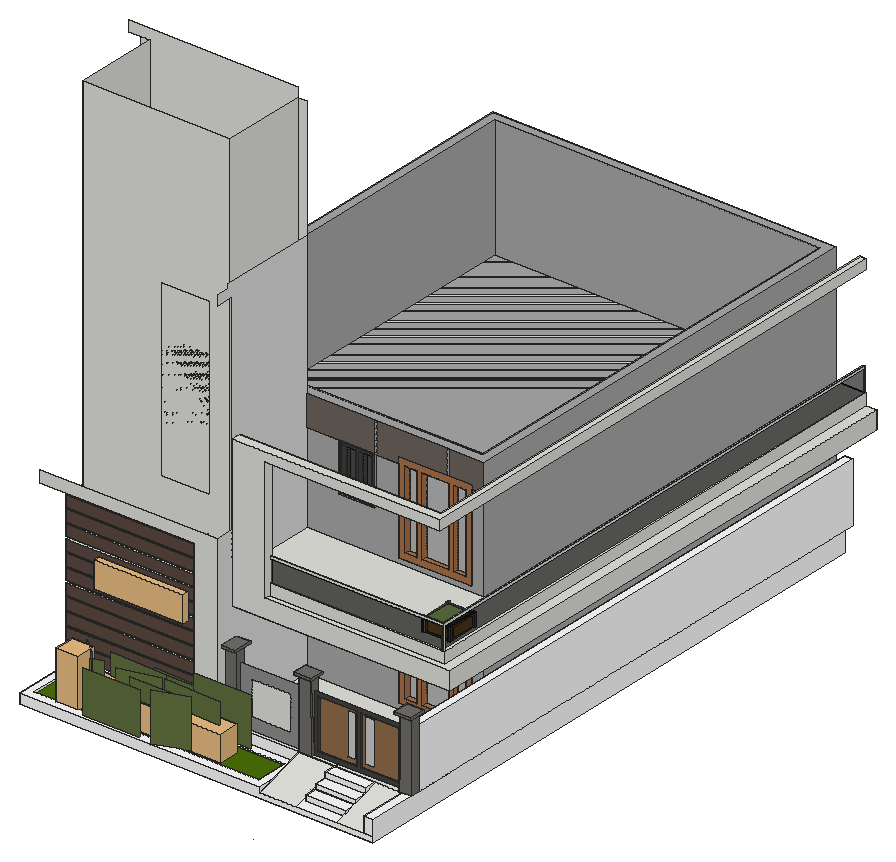
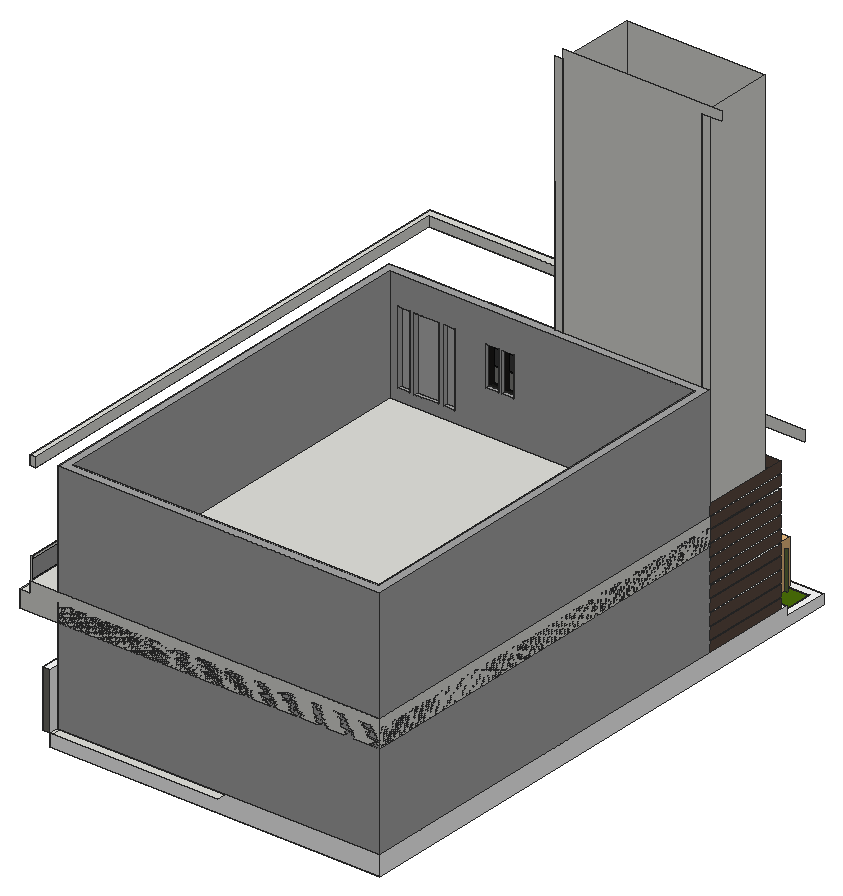
# SketchUp Ruby script. Lengths in inches.
U = 1.inch
M = Sketchup.active_model
def pt(a) = Geom::Point3d.new(a.map { |v| v * U })
def face(e, loops, mat)
  f = e.add_face(loops[0].map { |a| pt(a) })
  loops[1..].each { |l| e.add_face(l.map { |a| pt(a) }).erase! }
  f.material = f.back_material = mat if mat
  f
end
# faces: each face lists its corners as indices into pts; further lists are holes
def faces(e, pts, list, mat = nil) = list.each { |f| face(e, (f[0].is_a?(Array) ? f : [f]).map { |l| l.map { |i| pts[i] } }, mat) }
# xy, xz, yz: faces in a plane at the given z, y or x. An outline is a flat list of corners, or four numbers for a rectangle; further outlines are holes
def ring(l) = l.size == 4 ? [[l[0], l[1]], [l[2], l[1]], [l[2], l[3]], [l[0], l[3]]] : l.each_slice(2).to_a
def flat(e, list, mat, &to3) = list.each { |f| face(e, (f[0].is_a?(Array) ? f : [f]).map { |l| ring(l).map { |u, v| to3.(u, v) } }, mat) }
def xy(e, z, list, mat = nil) = flat(e, list, mat) { |x, y| [x, y, z] }
def xz(e, y, list, mat = nil) = flat(e, list, mat) { |x, z| [x, y, z] }
def yz(e, x, list, mat = nil) = flat(e, list, mat) { |y, z| [x, y, z] }
def lines(e, pts, list) = list.each { |a, b| e.add_line(pt(pts[a]), pt(pts[b])) }
# prism: a flat outline (further loops are holes) pulled along v
def prism(e, loops, v, mat = nil)
  f = face(e, loops, mat); d = Geom::Vector3d.new(v.map { |x| x * U })
  f.pushpull(f.normal.samedirection?(d) ? d.length : -d.length)
end
def box(e, o, s, mat = nil) = prism(e, [[o, [o[0] + s[0], o[1], o[2]], [o[0] + s[0], o[1] + s[1], o[2]], [o[0], o[1] + s[1], o[2]]]], [0, 0, s[2]], mat)
def at(x, y, z, deg = 0) = Geom::Transformation.translation(pt([x, y, z])) * Geom::Transformation.rotation(ORIGIN, Z_AXIS, deg.degrees)
def axes(o, x, y, z) = Geom::Transformation.new([*x, 0, *y, 0, *z, 0, *pt(o).to_a, 1])
def part(name) = M.definitions.add(name)
# library, detail: a bought-in or finely detailed component or shape, given as its bounding box
def library(name, o, s) = part(name).tap { |d| box(d.entities, o, s) }
def detail(e, o, s) = box(e.add_group.entities, o, s)
def put(e, d, t, mat = nil) = e.add_instance(d, t).tap { |i| i.material = mat if mat }
def group(e, t, mat = nil) = e.add_group.tap { |g| g.transformation = t; g.material = mat if mat }.entities
root = M.entities
M.materials.add("!长灌木1").color = [90, 107, 61]
M.materials.add("ARMANI GRIS").color = [109, 100, 95]
M.materials.add("Glass_Mirror_01").color = [185, 185, 185]
M.materials.add("Glass_Safety_01").color = [2, 2, 2]
M.materials["Glass_Safety_01"].alpha = 0.62
M.materials.add("Grass2").color = [97, 112, 61]
M.materials.add("M00_Soft_Cloud").color = [255, 255, 255]
M.materials.add("M01_Silver_Fog").color = [224, 224, 224]
M.materials.add("M03_Pewter_Shine").color = [168, 168, 168]
M.materials.add("M04_Stone_Frost").color = [142, 142, 142]
M.materials.add("Material20").color = [184, 138, 65]
M.materials.add("Material48").color = [126, 124, 110]
M.materials.add("Metal_Perforated_03_1K").color = [205, 205, 205]
M.materials.add("Roofing_04_1K").color = [112, 110, 103]
M.materials.add("Tile_Exterior_07_1K").color = [112, 111, 107]
M.materials.add("Wood_Floor_01_1K").color = [146, 111, 76]
M.materials.add("Wood_Floor_12_1K1").color = [92, 75, 65]
M.materials.add("Wood_Planks_01_1K").color = [69, 67, 63]
M.materials.add("Wood_Veneer_15_1K").color = [170, 114, 74]
M.materials.add("[Groundcover_BarkChips]").color = [80, 57, 35]
M.materials.add("[Groundcover_RiverRock_4inch]").color = [80, 57, 35]
M.materials.add("[Groundcover_Rock_Crushed_2inch]").color = [74, 111, 8]
c1 = part("Group\#22")
xz(c1.entities,0,[[0,0,62.37,62.37]],"Grass2")
c2 = part("Grass")
put(c2.entities,c1,at(102.75,113.61,7.86,-130.817))
put(c2.entities,c1,at(63.84,171.21,0.17))
put(c2.entities,c1,at(131.2,149.2,20.75))
put(c2.entities,c1,at(113.26,0,11.94,57.296))
put(c2.entities,c1,at(36.98,10.45,5.02))
put(c2.entities,c1,at(77.99,64.03,5.18))
put(c2.entities,c1,at(168.32,102.22,8.04,171.887))
put(c2.entities,c1,at(142.1,179.07,0,171.887))
put(c2.entities,c1,at(103.38,132.8,9.02,171.887))
put(c2.entities,c1,at(40.77,108.39,1.9,-130.817))
put(c2.entities,c1,at(14.86,142.73,10.93,-73.521))
c3 = part("Untitled")
xy(c3.entities,0.3125,[[-290.45,43.1875,-283.67,49.67]],"[Groundcover_RiverRock_4inch]")
xy(c3.entities,0.6875,[[-290.45,43.1875,-283.67,49.67]],"[Groundcover_Rock_Crushed_2inch]")
xz(c3.entities,43.1875,[[-290.45,0.3125,-283.67,0.6875]],"[Groundcover_BarkChips]")
xz(c3.entities,49.67,[[-290.45,0.3125,-283.67,0.6875]],"[Groundcover_BarkChips]")
yz(c3.entities,-290.45,[[43.1875,0.3125,49.67,0.6875]],"[Groundcover_BarkChips]")
yz(c3.entities,-283.67,[[43.1875,0.3125,49.67,0.6875]],"[Groundcover_BarkChips]")
c4 = library("Group_2",[-1.28,-0.39,0],[21.22,20.51,48.44])
c5 = library("Shrub planter",[0,0,0],[56.02,15.3,25.28])
c6 = library("WELCOMES  YOU  M",[0.16,0,0],[151.7,32.66,1])
c7 = part("组\#1")
xy(c7.entities,0,[[0,0,2.36,2.36],[29.92,0,32.28,2.36],[0,29.92,2.36,32.28],[29.92,29.92,32.28,32.28]],"Material48")
xy(c7.entities,1.57,[[2.36,0.39,2.36,2.36,0.39,2.36,0.39,29.92,2.36,29.92,2.36,31.89,29.92,31.89,29.92,29.92,31.89,29.92,31.89,2.36,29.92,2.36,29.92,0.39]],"Material48")
xy(c7.entities,2.76,[[3.54,0.39,28.74,1.57],[0.39,3.54,1.57,28.74],[30.71,3.54,31.89,28.74],[3.54,30.71,28.74,31.89]],"Material20")
xy(c7.entities,20.08,[[3.54,0.39,28.74,1.57],[0.39,3.54,1.57,28.74],[30.71,3.54,31.89,28.74],[3.54,30.71,28.74,31.89]],"Material20")
xy(c7.entities,21.0625,[[2.36,2.36,29.92,29.92]],"!长灌木1")
xy(c7.entities,21.26,[[2.36,0.39,29.92,2.36],[0.39,2.36,2.36,29.92],[29.92,2.36,31.89,29.92],[2.36,29.92,29.92,31.89]],"Material20")
xy(c7.entities,21.38,[[2.36,2.36,29.92,29.92]],"!长灌木1")
xy(c7.entities,22.83,[[0,0,2.36,2.36],[29.92,0,32.28,2.36],[0,29.92,2.36,32.28],[29.92,29.92,32.28,32.28]],"Material20")
xz(c7.entities,0,[[0,0,2.36,22.83],[29.92,0,32.28,22.83]],"Material20")
xz(c7.entities,0.39,[[[2.36,1.57,29.92,21.26],[3.54,2.76,28.74,20.08]]],"Material20")
xz(c7.entities,1.57,[[3.54,2.76,28.74,20.08]],"Material20")
xz(c7.entities,2.36,[[2.36,21.0625,29.92,21.38],[2.36,21.26,29.92,23.43]],"!长灌木1")
xz(c7.entities,2.36,[[0,0,0,22.83,2.36,22.83,2.36,21.26,0.39,21.26,0.39,1.57,2.36,1.57,2.36,0],[29.92,0,29.92,1.57,31.89,1.57,31.89,21.26,29.92,21.26,29.92,22.83,32.28,22.83,32.28,0]],"Material20")
xz(c7.entities,3.54,[[0.39,2.76,1.57,20.08],[30.71,2.76,31.89,20.08]],"Material20")
xz(c7.entities,28.74,[[0.39,2.76,1.57,20.08],[30.71,2.76,31.89,20.08]],"Material20")
xz(c7.entities,29.92,[[2.36,21.0625,29.92,21.38],[2.36,21.26,29.92,23.43]],"!长灌木1")
xz(c7.entities,29.92,[[0,0,2.36,0,2.36,1.57,0.39,1.57,0.39,22.83,0,22.83],[29.92,0,32.28,0,32.28,22.83,31.89,22.83,31.89,1.57,29.92,1.57],[0.39,21.26,2.36,22.83],[29.92,21.26,31.89,22.83]],"Material20")
xz(c7.entities,30.71,[[3.54,2.76,28.74,20.08]],"Material20")
xz(c7.entities,31.89,[[[2.36,1.57,29.92,21.26],[3.54,2.76,28.74,20.08]]],"Material20")
xz(c7.entities,32.28,[[0,0,2.36,22.83],[29.92,0,32.28,22.83]],"Material20")
yz(c7.entities,0,[[0,0,2.36,22.83],[29.92,0,32.28,22.83]],"Material20")
yz(c7.entities,0.39,[[[2.36,1.57,29.92,21.26],[3.54,2.76,28.74,20.08]]],"Material20")
yz(c7.entities,1.57,[[3.54,2.76,28.74,20.08]],"Material20")
yz(c7.entities,2.36,[[0,0,2.36,0,2.36,1.57,0.39,1.57,0.39,22.83,0,22.83]])
yz(c7.entities,2.36,[[2.36,21.0625,29.92,21.38],[2.36,21.26,29.92,23.43]],"!长灌木1")
yz(c7.entities,2.36,[[29.92,0,32.28,0,32.28,22.83,29.92,22.83,29.92,21.26,31.89,21.26,31.89,1.57,29.92,1.57],[0.39,21.26,2.36,22.83]],"Material20")
yz(c7.entities,3.54,[[0.39,2.76,1.57,20.08],[30.71,2.76,31.89,20.08]],"Material20")
yz(c7.entities,28.74,[[0.39,2.76,1.57,20.08],[30.71,2.76,31.89,20.08]],"Material20")
yz(c7.entities,29.92,[[2.36,21.0625,29.92,21.38],[2.36,21.26,29.92,23.43]],"!长灌木1")
yz(c7.entities,29.92,[[0,0,0,22.83,2.36,22.83,2.36,21.26,0.39,21.26,0.39,1.57,2.36,1.57,2.36,0],[29.92,0,29.92,1.57,31.89,1.57,31.89,21.26,29.92,21.26,29.92,22.83,32.28,22.83,32.28,0]],"Material20")
yz(c7.entities,30.71,[[3.54,2.76,28.74,20.08]],"Material20")
yz(c7.entities,31.89,[[[2.36,1.57,29.92,21.26],[3.54,2.76,28.74,20.08]]],"Material20")
yz(c7.entities,32.28,[[0,0,2.36,22.83],[29.92,0,32.28,22.83]],"Material20")
c8 = part("组\#2")
put(c8.entities,c7,at(24.1,23.99,0))
c9 = part("Potted tree")
put(c9.entities,c8,at(-24.1,-23.99,-1.57))
xy(root,0,[[153,39.125,177,57.125],[177,48.125,189,57.125],[189,48.125,250.64,52.625],[250.64,48.125,263.99,48.125,262.64,52.625,262.64,57.125,250.64,57.125],[263.99,48.125,350.58,48.125,351,52.625,262.64,52.625],
  [350.58,48.125,351.44,48.125,351.8,57.125,351,57.125,351,52.625],[351.44,48.125,363,48.125,363,57.125,351.8,57.125],[189,52.625,250.64,57.125],[262.64,52.625,351,57.125],[12,57.125,177,57.125,177,66.125,21,66.125,21,150.125,12,150.125],
  [177,57.125,351.8,66.125],[351.8,57.125,355.08,597.125],[355.08,57.125,363,597.125],[21,66.125,168,150.125],[168,66.125,177,150.125],
  [177,66.125,351.8,150.125],[177,150.125,351.8,597.125]])
xy(root,4,[[266.64,52.625,300.82,54.625],[300.82,52.625,304.82,54.625],[308.82,52.625,347,54.625]],"Wood_Planks_01_1K")
xy(root,11.02,[[12,57.125,153,57.125,153,58.16,13.04,58.16,13.04,150.125,12,150.125]])
xy(root,13.02,[[12,57.125,153,58.16],[12,58.16,13.04,150.125]])
xy(root,24.125,[[12,57.125,153,57.125,153,58.32,13.04,58.32,13.04,150.125,12,150.125]])
xy(root,26.125,[[12,57.125,153,58.32],[12,58.32,13.04,150.125]])
xy(root,37.22,[[12,57.125,153,57.125,153,59.125,14,59.125,14,150.125,12,150.125]])
xy(root,39.22,[[12,57.125,153,59.125],[12,59.125,14,150.125]])
xy(root,50.32,[[12,57.125,153,57.125,153,59.125,14,59.125,14,150.125,12,150.125]])
xy(root,52.32,[[12,57.125,153,59.125],[12,59.125,14,150.125]])
xy(root,53.75,[[266.64,52.625,300.82,54.625],[300.82,52.625,304.82,54.625],[308.82,52.625,347,54.625]],"Wood_Planks_01_1K")
xy(root,60,[[355.08,57.125,363,597.125]],"M00_Soft_Cloud")
xy(root,63.42,[[12,57.125,153,57.125,153,59.125,14,59.125,14,150.125,12,150.125]])
xy(root,65.42,[[12,57.125,153,59.125],[12,59.125,14,150.125]])
xy(root,69.65,[[177,43.125,177,48.125,189,48.125,189,57.125,177,57.125,177,62.125,191.48,62.125,191.48,43.125],[[348.24,44.71,365.25,61.2],[351,48.125,363,57.125]],[[248.05,45.06,265.59,59.96],[250.64,48.125,262.64,57.125]],[250.64,48.125,262.64,57.125],[351,48.125,363,57.125]])
xy(root,72,[[177,43.125,191.48,62.125],[348.24,44.71,365.25,61.2],[248.05,45.06,265.59,59.96]],"Tile_Exterior_07_1K")
xy(root,76.52,[[12,57.125,153,57.125,153,59.125,14,59.125,14,150.125,12,150.125]])
xy(root,78.52,[[12,57.125,153,59.125],[12,59.125,14,150.125]])
xy(root,89.62,[[12,57.125,153,57.125,153,59.125,14,59.125,14,150.125,12,150.125]])
xy(root,91.62,[[12,57.125,153,59.125],[12,59.125,14,150.125]])
xy(root,102.72,[[12,57.125,153,57.125,153,59.125,14,59.125,14,150.125,12,150.125]])
xy(root,104.72,[[12,57.125,153,59.125],[12,59.125,14,150.125]])
xy(root,115.82,[[12,57.125,153,57.125,153,59.125,14,59.125,14,150.125,12,150.125]])
xy(root,117.82,[[12,57.125,14,150.125],[14,57.125,153,59.125]])
xy(root,128.91,[[12,57.125,153,57.125,153,59.125,14,59.125,14,150.125,12,150.125]])
xy(root,130.91,[[12,57.125,14,150.125],[14,57.125,153,59.125]])
xz(root,39.125,[[153,0,177,0,177,168.01,0,168.01,0,156.01,153,156.01]])
xz(root,43.125,[[177,69.65,191.48,72]],"Tile_Exterior_07_1K")
xz(root,44.71,[[348.24,69.65,365.25,72]],"Tile_Exterior_07_1K")
xz(root,45.06,[[248.05,69.65,265.59,72]],"Tile_Exterior_07_1K")
xz(root,48.125,[[177,0,189,69.65],[250.64,0,263.99,0,262.64,69.65,250.64,69.65],[350.58,0,363,0,363,69.65,351,69.65,351,12]],"Tile_Exterior_07_1K")
xz(root,52.625,[[200.48,11.48,239.17,45.73]])
xz(root,52.625,[[[189,0,250.64,57.21],[200.48,11.48,239.17,45.73]]],"M04_Stone_Frost")
xz(root,52.625,[[[262.64,0,351,57.75],[266.64,4,304.82,53.75],[308.82,4,347,53.75]]],"Wood_Planks_01_1K")
xz(root,54.625,[[294.55,8.28,302.53,49.96],[312.36,8.28,320.34,49.96]],"Metal_Perforated_03_1K")
xz(root,54.625,[[[266.64,4,304.82,53.75],[294.55,8.28,302.53,49.96]],[[308.82,4,347,53.75],[312.36,8.28,320.34,49.96]]],"Wood_Floor_01_1K")
xz(root,57.125,[[351,0,351,69.65,363,69.65,363,60,355.08,60,355.08,0]],"Roofing_04_1K")
xz(root,57.125,[[177,0,189,69.65],[250.64,0,262.64,69.65]],"Tile_Exterior_07_1K")
xz(root,57.125,[[12,0,153,11.02],[12,13.02,153,24.125],[12,26.125,153,37.22],[12,39.22,153,50.32],[12,52.32,153,63.42],
  [12,65.42,153,76.52],[12,78.52,153,89.62],[12,91.62,153,102.72],[12,104.72,153,115.82],[12,117.82,153,128.91],
  [12,130.91,153,142.01]],"Wood_Floor_12_1K1")
xz(root,58.16,[[13.04,11.02,153,13.02]],"Wood_Planks_01_1K")
xz(root,58.32,[[13.04,24.125,153,26.125]],"Wood_Planks_01_1K")
xz(root,59.125,[[14,37.22,153,39.22],[14,50.32,153,52.32],[14,63.42,153,65.42],[14,76.52,153,78.52],[14,89.62,153,91.62],
  [14,102.72,153,104.72],[14,115.82,153,117.82],[14,128.91,153,130.91]],"Wood_Planks_01_1K")
xz(root,59.96,[[248.05,69.65,265.59,72]],"Tile_Exterior_07_1K")
xz(root,61.2,[[348.24,69.65,365.25,72]],"Roofing_04_1K")
xz(root,62.125,[[177,69.65,191.48,72]],"Tile_Exterior_07_1K")
xz(root,66.125,[[[21,0,168,510],[99.34,185.46,147.79,358.09]]])
xz(root,150.125,[[21,0,21,510,0,510,0,520,168,520,168,0],[12,0,12,11.02,13.04,11.02,13.04,13.02,12,13.02,12,24.125,13.04,24.125,13.04,26.125,12,26.125,12,37.22,14,37.22,14,39.22,12,39.22,12,50.32,14,50.32,14,52.32,12,52.32,12,63.42,14,63.42,14,65.42,12,65.42,12,76.52,14,76.52,14,78.52,12,78.52,12,89.62,14,89.62,14,91.62,12,91.62,12,102.72,14,102.72,14,104.72,12,104.72,12,115.82,14,115.82,14,117.82,12,117.82,12,128.91,14,128.91,14,130.91,12,130.91,12,142.01,14,142.01,14,144.01,12,144.01,12,510,21,510,21,0],[168,0,177,510]])
xz(root,597.125,[[355.08,0,363,60]],"Roofing_04_1K")
yz(root,12,[[57.125,0,150.125,11.02],[57.125,13.02,150.125,24.125],[57.125,26.125,150.125,37.22],[57.125,39.22,150.125,50.32],[57.125,52.32,150.125,63.42],
  [57.125,65.42,150.125,76.52],[57.125,78.52,150.125,89.62],[57.125,91.62,150.125,102.72],[57.125,104.72,150.125,115.82],[57.125,117.82,150.125,128.91],
  [57.125,130.91,150.125,142.01]],"Wood_Floor_12_1K1")
yz(root,13.04,[[58.16,11.02,150.125,13.02],[58.32,24.125,150.125,26.125]],"Wood_Planks_01_1K")
yz(root,14,[[59.125,37.22,150.125,39.22],[59.125,50.32,150.125,52.32],[59.125,63.42,150.125,65.42],[59.125,76.52,150.125,78.52],[59.125,89.62,150.125,91.62],
  [59.125,102.72,150.125,104.72],[59.125,115.82,150.125,117.82],[59.125,128.91,150.125,130.91]],"Wood_Planks_01_1K")
yz(root,21,[[66.125,0,150.125,510]])
yz(root,153,[[39.125,0,39.125,156.01,57.125,156.01,57.125,144.01,59.125,144.01,59.125,142.01,57.125,142.01,57.125,130.91,59.125,130.91,59.125,128.91,57.125,128.91,57.125,117.82,59.125,117.82,59.125,115.82,57.125,115.82,57.125,104.72,59.125,104.72,59.125,102.72,57.125,102.72,57.125,91.62,59.125,91.62,59.125,89.62,57.125,89.62,57.125,78.52,59.125,78.52,59.125,76.52,57.125,76.52,57.125,65.42,59.125,65.42,59.125,63.42,57.125,63.42,57.125,52.32,59.125,52.32,59.125,50.32,57.125,50.32,57.125,39.22,59.125,39.22,59.125,37.22,57.125,37.22,57.125,26.125,58.32,26.125,58.32,24.125,57.125,24.125,57.125,13.02,58.16,13.02,58.16,12,57.125,12,57.125,0],[57.125,11.02,58.16,12]])
yz(root,168,[[66.125,0,150.125,510]])
yz(root,177,[[39.125,0,48.125,0,48.125,69.65,43.125,69.65,43.125,72,62.125,72,62.125,69.65,57.125,69.65,57.125,0,150.125,0,150.125,390,52.125,390,52.125,386,39.125,386,39.125,376,57.125,376,57.125,168.01,39.125,168.01],[48.125,0,57.125,0,57.125,69.65,62.125,69.65,62.125,72,43.125,72,43.125,69.65,48.125,69.65]],"M01_Silver_Fog")
yz(root,189,[[48.125,0,57.125,69.65]],"Tile_Exterior_07_1K")
yz(root,191.48,[[43.125,69.65,62.125,72]],"Tile_Exterior_07_1K")
yz(root,248.05,[[45.06,69.65,59.96,72]],"Tile_Exterior_07_1K")
yz(root,250.64,[[0,-15,48.125,0,48.125,-15],[52.625,0,52.625,19.8,57.125,12,57.125,0]])
yz(root,250.64,[[48.125,0,48.125,12,52.625,19.8,52.625,0],[48.125,12,48.125,69.65,57.125,69.65,57.125,12,52.625,19.8]],"Tile_Exterior_07_1K")
yz(root,262.64,[[52.625,0,57.125,0,57.125,69.65,48.125,69.65]],"Tile_Exterior_07_1K")
yz(root,265.59,[[45.06,69.65,59.96,72]],"Tile_Exterior_07_1K")
yz(root,266.64,[[52.625,4,54.625,53.75]],"Wood_Planks_01_1K")
yz(root,304.82,[[52.625,4,54.625,53.75]],"Wood_Planks_01_1K")
yz(root,308.82,[[52.625,4,54.625,53.75]],"Wood_Planks_01_1K")
yz(root,347,[[52.625,4,54.625,13.44],[52.625,13.44,54.625,53.75]],"Wood_Planks_01_1K")
yz(root,348.24,[[44.71,69.65,61.2,72]],"Tile_Exterior_07_1K")
yz(root,351,[[52.625,0,52.625,13.44,57.125,12,57.125,0]])
yz(root,351,[[48.125,12,48.125,69.65,57.125,69.65,57.125,12,52.625,13.44]],"Tile_Exterior_07_1K")
yz(root,355.08,[[57.125,0,597.125,60]],"M00_Soft_Cloud")
yz(root,363,[[57.125,0,597.125,60]],"M00_Soft_Cloud")
yz(root,363,[[48.125,0,57.125,69.65]],"Roofing_04_1K")
yz(root,365.25,[[44.71,69.65,61.2,72]],"Tile_Exterior_07_1K")
p = [[250.64,48.125,0],[250.64,0,-15],[286.64,0,-15],[286.64,48.125,0],[263.99,48.125,0],[355.99,0,-15],
  [355.99,48.125,0],[351.44,48.125,0],[350.58,48.125,0],[327,48.125,0],[327,0,-15],[356.02,0,-15],
  [356.02,48.125,-15],[262.64,52.625,0],[262.64,48.125,69.65],[351,52.625,0],[351,52.625,13.44],[351,48.125,12],
  [286.27,-53.29,-20.63],[286.64,-53.29,-20.63],[286.64,17.48,-7.34],[286.64,17.6,-7.32]]
faces(root,p,[[0,1,2,3,4],[5,6,7,8,9,10],[6,11,12]])
faces(root,p,[[4,13,14],[15,8,16],[17,16,8]],"Tile_Exterior_07_1K")
lines(root,p,[[18,19],[20,21]])
put(root,c2,axes([38.67,0,-20],[0.91,0,0],[0,0.22562,0],[0,0,0.78]))
g1 = group(root,at(262.64,0,-20),"M00_Soft_Cloud")
xy(g1,0,[[-250.64,0,100.36,588.125]])
xy(g1,5,[[-12,0,91.09,0,91.09,57.125,24,57.125,24,48.125,-12,48.125],[-242.93,7.71,-19.71,40.41]])
xy(g1,10.5,[[[-250.64,0,-12,48.125],[-242.93,7.71,-19.71,40.41]]])
xy(g1,20,[[91.09,0,100.36,0,100.36,588.125,-250.64,588.125,-250.64,48.125,24,48.125,24,57.125,91.09,57.125]])
xz(g1,0,[[-250.64,0,-250.64,10.5,-12,10.5,-12,5,100.36,5,100.36,0],[91.09,5,100.36,20]])
xz(g1,7.71,[[-242.93,5,-19.71,10.5]])
xz(g1,40.41,[[-242.93,5,-19.71,10.5]])
xz(g1,48.125,[[-12,5,24,5,24,20,-250.64,20,-250.64,10.5,-12,10.5]])
xz(g1,57.125,[[24,5,91.09,20]])
xz(g1,588.125,[[-250.64,0,100.36,20]])
yz(g1,-250.64,[[0,0,588.125,0,588.125,20,48.125,20,48.125,10.5,0,10.5]])
yz(g1,-242.93,[[7.71,5,40.41,10.5]])
yz(g1,-19.71,[[7.71,5,40.41,10.5]])
yz(g1,-12,[[0,5,48.125,10.5]])
yz(g1,24,[[48.125,5,57.125,20]])
yz(g1,91.09,[[0,5,57.125,20]])
yz(g1,100.36,[[0,0,588.125,20]])
p = [[24,12.03,5],[24,48.125,5]]
lines(g1,p,[[0,1]])
put(root,c3,axes([9623.06,-219.625,-19.32],[33.07002,0,0],[0,5.25447,0],[0,0,12.13758]))
g2 = group(root,at(262.64,12.03,-15),"M00_Soft_Cloud")
box(g2,[24,0,0],[40.36,12.03,5])
put(root,c4,at(43.39,7.29,-10.97))
put(root,c5,axes([69.27,12.15,-10.97],[2.36,0,0],[0,1.37,0],[0,0,1]))
g3 = group(root,at(262.64,24.0625,-10),"M00_Soft_Cloud")
box(g3,[24,0,0],[40.36,12.03,5])
g4 = group(root,at(262.64,36.09,-5),"M00_Soft_Cloud")
xy(g4,0,[[24,0,64.36,12.03]])
xy(g4,5,[[24,0,64.36,12.03]])
xz(g4,0,[[24,0,64.36,5]],"M00_Soft_Cloud")
xz(g4,12.03,[[24,0,64.36,5]])
yz(g4,24,[[0,0,12.03,5]])
yz(g4,64.36,[[0,0,12.03,5]])
g5 = group(root,at(12,150.125,0),"M03_Pewter_Shine")
xy(g5,0,[[9,9,333,429]])
xy(g5,6,[[258,-1,330,0]])
xy(g5,12,[[264,4.5,276,9],[281,4.5,307,9],[312,4.5,324,9]])
xy(g5,12,[[264,-1,276,4.5],[281,-1,307,4.5],[312,-1,324,4.5]],"Wood_Veneer_15_1K")
xy(g5,42,[[198,-1,234,0]])
xy(g5,45,[[201,4.5,214.5,9],[217.5,4.5,231,9]])
xy(g5,45,[[201,-1,214.5,4.5],[217.5,-1,231,4.5]],"Wood_Planks_01_1K")
xy(g5,87,[[201,4.5,214.5,9],[217.5,4.5,231,9]])
xy(g5,87,[[201,-1,214.5,4.5],[217.5,-1,231,4.5]],"Wood_Planks_01_1K")
xy(g5,90,[[198,-1,234,0],[264,4.5,276,9],[281,4.5,307,9],[312,4.5,324,9]])
xy(g5,90,[[264,-1,276,4.5],[281,-1,307,4.5],[312,-1,324,4.5]],"Wood_Veneer_15_1K")
xy(g5,96,[[258,-1,330,0]])
xy(g5,120,[[[0,0,342,438],[9,9,333,429]]])
xz(g5,-1,[[[198,42,234,90],[199.48,43.48,232.52,88.52]]])
xz(g5,-1,[[[199.48,43.48,232.52,88.52],[201,45,214.5,87],[217.5,45,231,87]]],"Wood_Planks_01_1K")
xz(g5,-1,[[[258,6,330,96],[281,12,307,90],[264,12,276,90],[312,12,324,90]]],"Wood_Veneer_15_1K")
xz(g5,0,[[0,0,9,120],[9,0,156,120],[156,0,165,120],[[165,0,342,120],[258,6,330,96],[198,42,234,90]]])
xz(g5,4.5,[[264,12,276,90],[281,12,307,90],[312,12,324,90]],"Glass_Mirror_01")
xz(g5,4.5,[[201,45,214.5,87],[217.5,45,231,87]],"Glass_Safety_01")
xz(g5,9,[[[9,0,333,120],[281,12,307,90],[264,12,276,90],[312,12,324,90],[201,45,214.5,87],[217.5,45,231,87]]])
xz(g5,429,[[9,0,333,120]])
xz(g5,438,[[0,0,342,120]])
yz(g5,0,[[0,0,438,120]])
yz(g5,9,[[9,0,429,120]])
yz(g5,198,[[-1,42,0,90]])
yz(g5,201,[[4.5,45,9,87]])
yz(g5,201,[[-1,45,4.5,87]],"Wood_Planks_01_1K")
yz(g5,214.5,[[4.5,45,9,87]])
yz(g5,214.5,[[-1,45,4.5,87]],"Wood_Planks_01_1K")
yz(g5,217.5,[[4.5,45,9,87]])
yz(g5,217.5,[[-1,45,4.5,87]],"Wood_Planks_01_1K")
yz(g5,231,[[4.5,45,9,87]])
yz(g5,231,[[-1,45,4.5,87]],"Wood_Planks_01_1K")
yz(g5,234,[[-1,42,0,90]])
yz(g5,258,[[-1,6,0,96]])
yz(g5,264,[[4.5,12,9,90]])
yz(g5,264,[[-1,12,4.5,90]],"Wood_Veneer_15_1K")
yz(g5,276,[[4.5,12,9,90]])
yz(g5,276,[[-1,12,4.5,90]],"Wood_Veneer_15_1K")
yz(g5,281,[[4.5,12,9,90]])
yz(g5,281,[[-1,12,4.5,90]],"Wood_Veneer_15_1K")
yz(g5,307,[[4.5,12,9,90]])
yz(g5,307,[[-1,12,4.5,90]],"Wood_Veneer_15_1K")
yz(g5,312,[[4.5,12,9,90]])
yz(g5,312,[[-1,12,4.5,90]],"Wood_Veneer_15_1K")
yz(g5,324,[[4.5,12,9,90]])
yz(g5,324,[[-1,12,4.5,90]],"Wood_Veneer_15_1K")
yz(g5,330,[[-1,6,0,96]])
yz(g5,333,[[9,0,429,120]])
yz(g5,342,[[0,0,438,120]])
put(root,c6,axes([44.85,57.125,72.28],[0.58198,0,0],[0,0,0.79],[0,-6.272,0]),"M00_Soft_Cloud")
g6 = group(root,at(12,150.125,120))
xy(g6,-19,[[[165,-93,165,0,0,0,0,438,382,438,382,-93],[177,-72,360,-72,360,426,12,426,12,12,177,12]]])
xy(g6,-1,[[198,-93,382,-93,382,438,372,438,372,-87.2,198,-87.2]])
xy(g6,0,[[177,-72,177,12,12,12,12,426,360,426,360,-72]])
xy(g6,10,[[[198,-87.2,372,-87.2,372,438,0,438,0,0,165,0,165,-84,198,-84,198,-86.21,369.28,-86.21,369.28,-85.81,371.07,-85.81,371.07,-86.61,369.28,-86.61,369.28,-86.21,198,-86.21],[370.66,436.68,371.33,437.5]]])
xy(g6,32,[[153.21,-86.61,198,-85.81],[198,-86.61,369.28,-86.21],[198,-86.21,369.28,-85.81],[369.28,-85.81,370.34,436.4],[370.34,-85.81,371.07,436.4]])
xy(g6,34,[[153.21,-86.61,371.07,-86.61,371.07,436.4,369.28,436.4,369.28,-85.81,153.21,-85.81],[370.66,436.68,371.33,437.5]])
xy(g6,120.32,[[198,-93,198,-84,366,-84,366,438,372,438,372,-93]])
xy(g6,130,[[165,-93,372,-93,372,438,366,438,366,-84,165,-84]])
xz(g6,-93,[[165,-19,382,-19,382,-1,198,-1,198,120.32,372,120.32,372,130,165,130]])
xz(g6,-87.2,[[198,-1,372,10]])
xz(g6,-86.61,[[369.28,10,371.07,10,371.07,34,153.21,34,153.21,32,369.28,32]])
xz(g6,-86.21,[[198,10,369.28,32]],"Glass_Safety_01")
xz(g6,-85.81,[[369.28,10,370.34,32],[370.34,10,371.07,32],[153.21,32,369.28,34]])
xz(g6,-84,[[165,10,165,130,366,130,366,120.32,198,120.32,198,10]])
xz(g6,-72,[[177,-19,360,0]])
xz(g6,0,[[0,-19,165,10]])
xz(g6,12,[[12,-19,177,0]])
xz(g6,426,[[12,-19,360,0]])
xz(g6,436.4,[[369.28,32,371.07,34]])
xz(g6,436.68,[[370.66,10,371.33,34]])
xz(g6,437.5,[[370.66,10,371.33,34]])
xz(g6,438,[[0,-19,0,10,372,10,372,-1,382,-1,382,-19],[366,120.32,372,130]])
yz(g6,0,[[0,-19,438,10]])
yz(g6,12,[[12,-19,426,0]])
yz(g6,153.21,[[-86.61,32,-85.81,34]])
yz(g6,165,[[-93,-19,-93,130,-84,130,-84,10,0,10,0,-19]])
yz(g6,177,[[-72,-19,12,0]])
yz(g6,198,[[-93,-1,-87.2,-1,-87.2,10,-84,10,-84,120.32,-93,120.32]])
yz(g6,360,[[-72,-19,426,0]])
yz(g6,366,[[-84,120.32,438,130]])
yz(g6,369.28,[[-86.61,10,-86.21,32],[-86.21,10,-85.81,32],[-85.81,32,436.4,34]])
yz(g6,370.66,[[436.68,10,437.5,34]])
yz(g6,371.07,[[-86.61,10,-85.81,10,-85.81,32,436.4,32,436.4,34,-86.61,34]])
yz(g6,371.33,[[436.68,10,437.5,34]])
yz(g6,372,[[-87.2,-1,438,10],[-93,120.32,438,130]])
yz(g6,382,[[-93,-19,438,-1]])
p = [[370.34,-85.81,32],[370.34,-85.81,10],[371.02,436.4,10],[371.02,436.4,32],[371.02,436.4,32.02],[370.34,-85.81,32.02],
  [198,-85.81,32],[198,-85.8,32]]
faces(g6,p,[[0,1,2,3,4,5]],"Glass_Safety_01")
lines(g6,p,[[6,7]])
put(root,c9,axes([349.98,77.78,130],[0.87,0,0],[0,1,0],[0,0,0.60829]))
g7 = group(root,at(12,150.125,130),"M03_Pewter_Shine")
xy(g7,0,[[9,9,333,429]])
xy(g7,6,[[258,-1,330,0]])
xy(g7,12,[[264,4.5,276,9],[281,4.5,307,9],[312,4.5,324,9]])
xy(g7,12,[[264,-1,276,4.5],[281,-1,307,4.5],[312,-1,324,4.5]],"Wood_Veneer_15_1K")
xy(g7,42,[[198,-1,234,0]])
xy(g7,45,[[201,4.5,214.5,9],[217.5,4.5,231,9]])
xy(g7,45,[[201,-1,214.5,4.5],[217.5,-1,231,4.5]],"Wood_Planks_01_1K")
xy(g7,87,[[201,4.5,214.5,9],[217.5,4.5,231,9]])
xy(g7,87,[[201,-1,214.5,4.5],[217.5,-1,231,4.5]],"Wood_Planks_01_1K")
xy(g7,90,[[165,-1,198,0],[234,-1,258,0],[264,4.5,276,9],[281,4.5,307,9],[312,4.5,324,9]])
xy(g7,90,[[264,-1,276,4.5],[281,-1,307,4.5],[312,-1,324,4.5]],"Wood_Veneer_15_1K")
xy(g7,92.5625,[[330,-1,342,0]])
xy(g7,120,[[[165,-1,342,-1,342,438,0,438,0,0,165,0],[9,9,333,429]]])
xz(g7,-1,[[[198,42,234,90],[199.48,43.48,232.52,88.52]],[234,90,236,120],[304.99,96,306.99,120]])
xz(g7,-1,[[165,90,234,120],[236,90,258,90,258,96,304.99,96,304.99,120,236,120],[330,92.5625,342,92.5625,342,120,306.99,120,306.99,96,330,96]],"ARMANI GRIS")
xz(g7,-1,[[[199.48,43.48,232.52,88.52],[201,45,214.5,87],[217.5,45,231,87]]],"Wood_Planks_01_1K")
xz(g7,-1,[[[258,6,330,96],[281,12,307,90],[264,12,276,90],[312,12,324,90]]],"Wood_Veneer_15_1K")
xz(g7,0,[[0,0,9,120],[9,0,156,120],[156,0,165,120],[165,0,342,0,342,92.5625,330,92.5625,330,6,258,6,258,90,234,90,234,42,198,42,198,90,165,90]])
xz(g7,4.5,[[264,12,276,90],[281,12,307,90],[312,12,324,90]],"Glass_Mirror_01")
xz(g7,4.5,[[201,45,214.5,87],[217.5,45,231,87]],"Glass_Safety_01")
xz(g7,9,[[[9,0,333,120],[281,12,307,90],[264,12,276,90],[312,12,324,90],[201,45,214.5,87],[217.5,45,231,87]]])
xz(g7,429,[[9,0,333,120]])
xz(g7,438,[[0,0,342,120]])
yz(g7,0,[[0,0,438,120]])
yz(g7,9,[[9,0,429,120]])
yz(g7,165,[[-1,90,0,105],[-1,105,0,120]])
yz(g7,198,[[-1,42,0,90]])
yz(g7,201,[[4.5,45,9,87]])
yz(g7,201,[[-1,45,4.5,87]],"Wood_Planks_01_1K")
yz(g7,214.5,[[4.5,45,9,87]])
yz(g7,214.5,[[-1,45,4.5,87]],"Wood_Planks_01_1K")
yz(g7,217.5,[[4.5,45,9,87]])
yz(g7,217.5,[[-1,45,4.5,87]],"Wood_Planks_01_1K")
yz(g7,231,[[4.5,45,9,87]])
yz(g7,231,[[-1,45,4.5,87]],"Wood_Planks_01_1K")
yz(g7,234,[[-1,42,0,90]])
yz(g7,258,[[-1,6,0,90]])
yz(g7,264,[[4.5,12,9,90]])
yz(g7,264,[[-1,12,4.5,90]],"Wood_Veneer_15_1K")
yz(g7,276,[[4.5,12,9,90]])
yz(g7,276,[[-1,12,4.5,90]],"Wood_Veneer_15_1K")
yz(g7,281,[[4.5,12,9,90]])
yz(g7,281,[[-1,12,4.5,90]],"Wood_Veneer_15_1K")
yz(g7,307,[[4.5,12,9,90]])
yz(g7,307,[[-1,12,4.5,90]],"Wood_Veneer_15_1K")
yz(g7,312,[[4.5,12,9,90]])
yz(g7,312,[[-1,12,4.5,90]],"Wood_Veneer_15_1K")
yz(g7,324,[[4.5,12,9,90]])
yz(g7,324,[[-1,12,4.5,90]],"Wood_Veneer_15_1K")
yz(g7,330,[[-1,6,0,92.5625]])
yz(g7,333,[[9,0,429,120]])
yz(g7,342,[[0,0,438,0,438,120,-1,120,-1,92.5625,0,92.5625]])
